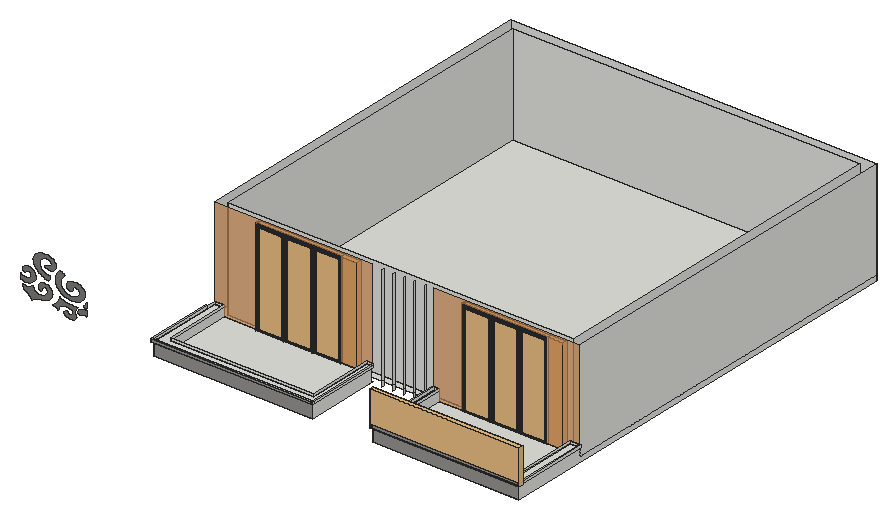
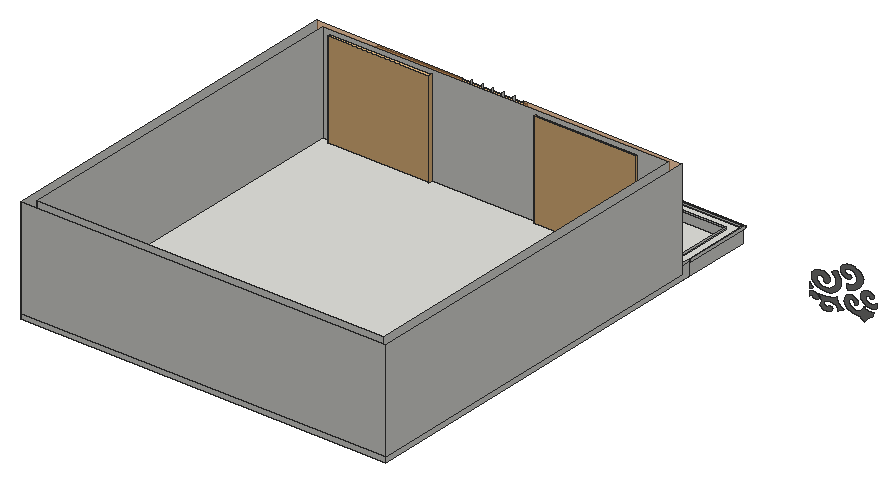
# SketchUp Ruby script. Lengths in inches.
U = 1.inch
M = Sketchup.active_model
def pt(a) = Geom::Point3d.new(a.map { |v| v * U })
def face(e, loops, mat)
  f = e.add_face(loops[0].map { |a| pt(a) })
  loops[1..].each { |l| e.add_face(l.map { |a| pt(a) }).erase! }
  f.material = f.back_material = mat if mat
  f
end
# faces: each face lists its corners as indices into pts; further lists are holes
def faces(e, pts, list, mat = nil) = list.each { |f| face(e, (f[0].is_a?(Array) ? f : [f]).map { |l| l.map { |i| pts[i] } }, mat) }
# xy, xz, yz: faces in a plane at the given z, y or x. An outline is a flat list of corners, or four numbers for a rectangle; further outlines are holes
def ring(l) = l.size == 4 ? [[l[0], l[1]], [l[2], l[1]], [l[2], l[3]], [l[0], l[3]]] : l.each_slice(2).to_a
def flat(e, list, mat, &to3) = list.each { |f| face(e, (f[0].is_a?(Array) ? f : [f]).map { |l| ring(l).map { |u, v| to3.(u, v) } }, mat) }
def xy(e, z, list, mat = nil) = flat(e, list, mat) { |x, y| [x, y, z] }
def xz(e, y, list, mat = nil) = flat(e, list, mat) { |x, z| [x, y, z] }
def yz(e, x, list, mat = nil) = flat(e, list, mat) { |y, z| [x, y, z] }
def lines(e, pts, list) = list.each { |a, b| e.add_line(pt(pts[a]), pt(pts[b])) }
# prism: a flat outline (further loops are holes) pulled along v
def prism(e, loops, v, mat = nil)
  f = face(e, loops, mat); d = Geom::Vector3d.new(v.map { |x| x * U })
  f.pushpull(f.normal.samedirection?(d) ? d.length : -d.length)
end
def box(e, o, s, mat = nil) = prism(e, [[o, [o[0] + s[0], o[1], o[2]], [o[0] + s[0], o[1] + s[1], o[2]], [o[0], o[1] + s[1], o[2]]]], [0, 0, s[2]], mat)
def at(x, y, z, deg = 0) = Geom::Transformation.translation(pt([x, y, z])) * Geom::Transformation.rotation(ORIGIN, Z_AXIS, deg.degrees)
def axes(o, x, y, z) = Geom::Transformation.new([*x, 0, *y, 0, *z, 0, *pt(o).to_a, 1])
def part(name) = M.definitions.add(name)
# library, detail: a bought-in or finely detailed component or shape, given as its bounding box
def library(name, o, s) = part(name).tap { |d| box(d.entities, o, s) }
def detail(e, o, s) = box(e.add_group.entities, o, s)
def put(e, d, t, mat = nil) = e.add_instance(d, t).tap { |i| i.material = mat if mat }
def group(e, t, mat = nil) = e.add_group.tap { |g| g.transformation = t; g.material = mat if mat }.entities
root = M.entities
M.materials.add("Wine2").color = [0, 0, 0]
M.materials["Wine2"].alpha = 0
M.materials.add("[0043_SaddleBrown]4").color = [124, 123, 122]
M.materials.add("[0130_Gainsboro]").color = [39, 45, 50]
M.materials.add("[Granite Light Gray]").color = [149, 148, 144]
M.materials.add("[Wood Floor Light]").color = [204, 176, 127]
M.materials.add("[Wood Floor]").color = [224, 152, 88]
M.materials["[Wood Floor]"].alpha = 0.68
c1 = part("Framed glazing panel")
xy(c1.entities,0,[[0,-0.98,43.07,0],[0,0,43.07,1.4]],"[0130_Gainsboro]")
xy(c1.entities,0.3,[[0.3,-1.43,42.77,-0.98]],"[0130_Gainsboro]")
xy(c1.entities,2.95,[[2.95,-1.43,40.12,-0.63],[2.95,-0.63,40.12,0],[2.95,0,40.12,0.64],[2.95,0.64,40.12,1.4]],"[0130_Gainsboro]")
xy(c1.entities,3.54,[[3.54,-0.63,39.53,0],[3.54,0,39.53,0.64]],"[0130_Gainsboro]")
xy(c1.entities,111.8125,[[3.54,-0.63,39.53,0],[3.54,0,39.53,0.64]],"[0130_Gainsboro]")
xy(c1.entities,112.4,[[2.95,-1.43,40.12,-0.63],[2.95,-0.63,40.12,0],[2.95,0,40.12,0.64],[2.95,0.64,40.12,1.4]],"[0130_Gainsboro]")
xy(c1.entities,115.05,[[0.3,-1.43,42.77,-0.98]],"[0130_Gainsboro]")
xy(c1.entities,115.35,[[0,-0.98,43.07,0],[0,0,43.07,1.4]],"[0130_Gainsboro]")
xz(c1.entities,-1.43,[[[0.3,0.3,42.77,115.05],[2.95,2.95,40.12,112.4]]],"[0130_Gainsboro]")
xz(c1.entities,-0.98,[[[0,0,43.07,115.35],[0.3,0.3,42.77,115.05]]],"[0130_Gainsboro]")
xz(c1.entities,-0.63,[[[2.95,2.95,40.12,112.4],[3.54,3.54,39.53,111.8125]]],"[0130_Gainsboro]")
xz(c1.entities,0,[[3.54,3.54,39.53,111.8125]],"Wine2")
xz(c1.entities,0,[[[0,0,43.07,115.35],[2.95,2.95,40.12,112.4]],[[2.95,2.95,40.12,112.4],[3.54,3.54,39.53,111.8125]]],"[0130_Gainsboro]")
xz(c1.entities,0.64,[[[2.95,2.95,40.12,112.4],[3.54,3.54,39.53,111.8125]]],"[0130_Gainsboro]")
xz(c1.entities,1.4,[[[0,0,43.07,115.35],[2.95,2.95,40.12,112.4]]],"[0130_Gainsboro]")
yz(c1.entities,0,[[-0.98,0,0,115.35],[0,0,1.4,115.35]],"[0130_Gainsboro]")
yz(c1.entities,0.3,[[-1.43,0.3,-0.98,115.05]],"[0130_Gainsboro]")
yz(c1.entities,2.95,[[-1.43,2.95,-0.63,112.4],[-0.63,2.95,0,112.4],[0,2.95,0.64,112.4],[0.64,2.95,1.4,112.4]],"[0130_Gainsboro]")
yz(c1.entities,3.54,[[-0.63,3.54,0,111.8125],[0,3.54,0.64,111.8125]],"[0130_Gainsboro]")
yz(c1.entities,39.53,[[-0.63,3.54,0,111.8125],[0,3.54,0.64,111.8125]],"[0130_Gainsboro]")
yz(c1.entities,40.12,[[-1.43,2.95,-0.63,112.4],[-0.63,2.95,0,112.4],[0,2.95,0.64,112.4],[0.64,2.95,1.4,112.4]],"[0130_Gainsboro]")
yz(c1.entities,42.77,[[-1.43,0.3,-0.98,115.05]],"[0130_Gainsboro]")
yz(c1.entities,43.07,[[-0.98,0,0,115.35],[0,0,1.4,115.35]],"[0130_Gainsboro]")
c2 = part("Glazing assembly")
put(c2.entities,c1,axes([90.57,1.43,0],[1.05148,0,0],[0,1,0],[0,0,1]))
put(c2.entities,c1,axes([0,1.43,0],[1.05148,0,0],[0,1,0],[0,0,1]))
put(c2.entities,c1,axes([45.29,1.43,0],[1.05148,0,0],[0,1,0],[0,0,1]))
c3 = library("Curtains",[0,0,0],[121.73,8.19,117.22])
c4 = library("Glass Railing",[0,0,0],[139.5,4.76,42])
xy(root,388.875,[[3103.26,651.03,3204.51,657.03],[3351.01,651.03,3452.26,657.03]])
xy(root,394.4375,[[3053.01,559.875,3243.69,570.83],[3316.14,559.875,3491.44,570.83],[3064.33,657.03,3480.11,1085.17]])
xy(root,394.4375,[[3053.01,570.83,3064.33,651.03],[3064.33,570.83,3243.69,651.03],[3316.14,570.83,3480.11,651.03],[3480.11,570.83,3491.44,651.03]],"[Wood Floor Light]")
xy(root,400.4375,[[3064.33,570.83,3235.84,570.83,3235.84,651.03,3204.51,651.03,3204.51,657.03,3103.26,657.03,3103.26,651.03,3064.33,651.03],[3322.22,570.83,3480.11,570.83,3480.11,651.03,3452.26,651.03,3452.26,657.03,3351.01,657.03,3351.01,651.03,3322.22,651.03],[3053.01,651.03,3053.01,1096.5,3491.44,1096.5,3491.44,651.03,3452.26,651.03,3452.26,657.03,3480.11,657.03,3480.11,1085.17,3064.33,1085.17,3064.33,657.03,3103.26,657.03,3103.26,651.03],[3064.33,657.03,3480.11,1085.17]])
xy(root,410.625,[[3051.26,557.9375,3243.69,559.875],[3243.69,557.9375,3245.63,559.875],[3314.21,557.9375,3316.14,559.875],[3316.14,557.9375,3491.44,559.875],[3491.44,557.9375,3493.37,559.875],
  [3051.07,559.875,3053.01,640.11],[3053.01,559.875,3053.01,651.03,3064.33,651.03,3064.33,570.83,3235.84,570.83,3235.84,651.03,3243.69,651.03,3243.69,559.875],[3243.69,559.875,3245.63,647.91],[3314.21,559.875,3316.14,651.03],[3316.14,559.875,3316.14,651.03,3322.22,651.03,3322.22,570.83,3480.11,570.83,3480.11,651.03,3491.44,651.03,3491.44,559.875],
  [3491.44,559.875,3493.37,651.03]])
xz(root,557.9375,[[3491.44,410.625,3493.37,413.5]])
xz(root,557.9375,[[3051.26,410.625,3243.69,413.5],[3243.69,410.625,3245.63,413.5],[3314.21,410.625,3316.14,413.5],[3316.14,410.625,3491.44,413.5]],"[Granite Light Gray]")
xz(root,559.875,[[3051.07,410.625,3051.26,413.5],[3051.26,410.625,3053.01,413.5],[3053.01,410.625,3243.69,413.5],[3243.69,410.625,3245.63,413.5],[3314.21,410.625,3316.14,413.5],
  [3316.14,410.625,3491.44,413.5],[3491.44,410.625,3493.37,413.5]])
xz(root,559.875,[[3053.01,394.4375,3243.69,410.625],[3316.14,394.4375,3491.44,410.625]],"[Granite Light Gray]")
xz(root,570.83,[[3064.33,400.4375,3235.84,410.625],[3322.22,400.4375,3480.11,410.625],[3064.33,410.625,3235.84,413.5],[3322.22,410.625,3480.11,413.5]])
xz(root,589.17,[[2928.78,378.34,2930.4375,378.37,2932.06,378.64,2933.5625,379.15,2934.89,379.86,2935.99,380.76,2936.81,381.8,2936.25,382.74,2935.8,383.71,2935.48,384.71,2935.28,385.72,2935.2,386.75,2935.25,387.77,2935.43,388.79,2935.73,389.79,2936.15,390.76,2936.69,391.71,2937.35,392.62,2938.11,393.48,2936.23,393.37,2934.35,393.33,2932.46,393.38,2930.59,393.5,2928.72,393.71,2926.88,393.99,2925.06,394.35,2923.27,394.79,2921.53,395.3,2919.82,395.88,2918.17,396.54,2916.57,397.26,2916.46,396.19,2916.23,395.13,2915.89,394.09,2915.44,393.07,2914.89,392.07,2914.24,391.11,2913.49,390.1875,2912.64,389.31,2911.71,388.47,2910.6875,387.69,2909.59,386.97,2908.42,386.31,2909.04,386.1,2909.65,385.89,2910.26,385.67,2910.86,385.44,2911.45,385.2,2912.04,384.95,2912.62,384.7,2913.19,384.44,2913.75,384.16,2914.3125,383.88,2914.86,383.59,2915.4,383.3,2915.51,384.7,2916.03,386.05,2916.95,387.29,2918.23,388.35,2919.79,389.19,2921.57,389.77,2923.47,390.05,2925.42,390.03,2927.32,389.7,2929.07,389.08,2930.59,388.2,2931.81,387.11,2931.85,386.77,2931.87,386.43,2931.87,385.75,2931.81,385.07,2931.76,384.73,2931.69,384.39,2931.61,384.06,2931.52,383.72,2931.42,383.39,2931.29,383.06,2930.7,382.875,2930.07,382.76,2929.43,382.72,2928.78,382.75,2928.15,382.85,2927.55,383.03,2927,383.27,2926.5,383.58,2926.08,383.93,2925.75,384.33,2925.5,384.76,2925.36,385.22,2924.95,385.09,2924.5625,384.95,2924.18,384.79,2923.82,384.61,2923.47,384.41,2923.14,384.2,2922.83,383.98,2922.53,383.74,2922.26,383.48,2922.02,383.22,2921.79,382.95,2921.59,382.66,2922.18,381.54,2923.07,380.53,2924.23,379.68,2925.61,379.01,2927.14,378.55],[2883.21,382.25,2883.82,383.03,2884.54,383.77,2885.35,384.44,2886.26,385.06,2887.25,385.6,2888.3125,386.07,2889.44,386.46,2890.61,386.77,2891.82,386.98,2893.05,387.11,2894.29,387.15,2895.54,387.09,2897.95,387.5,2900.24,388.2,2902.32,389.18,2904.125,390.4,2905.61,391.84,2906.73,393.4375,2907.44,395.15,2907.73,396.93,2907.58,398.71,2907.01,400.46,2906.02,402.1,2904.65,403.59,2903.52,404.41,2902.18,405.05,2900.68,405.47,2899.09,405.65,2897.49,405.59,2895.9375,405.29,2894.51,404.75,2893.27,404.02,2892.27,403.11,2891.56,402.07,2891.16,400.95,2891.11,399.79,2891.17,399.43,2891.28,399.08,2891.44,398.73,2891.65,398.4,2891.91,398.09,2892.21,397.8,2892.55,397.53,2892.92,397.29,2893.33,397.08,2893.77,396.9,2894.23,396.75,2894.71,396.64,2894.79,397.15,2894.91,397.65,2895.07,398.15,2895.28,398.64,2895.52,399.13,2895.8,399.6,2896.12,400.06,2896.48,400.5,2896.87,400.93,2897.29,401.34,2897.75,401.74,2898.24,402.11,2899.17,401.77,2900.02,401.34,2900.77,400.81,2901.4,400.2,2901.89,399.54,2902.23,398.83,2902.42,398.08,2902.44,397.33,2902.3,396.58,2902.01,395.86,2901.57,395.18,2900.98,394.55,2900.14,393.61,2899.07,392.8,2897.82,392.14,2896.42,391.66,2894.92,391.38,2893.37,391.3,2891.83,391.43,2890.34,391.76,2888.97,392.28,2887.76,392.98,2886.74,393.82,2885.96,394.79,2885.74,395.05,2885.54,395.3125,2885.35,395.58,2885.17,395.85,2885,396.13,2884.85,396.41,2884.71,396.69,2884.58,396.98,2884.47,397.27,2884.36,397.5625,2884.27,397.86,2884.2,398.15,2883.51,397.49,2882.71,396.89,2881.81,396.375,2880.83,395.94,2879.78,395.6,2878.6875,395.35,2877.55,395.2,2876.41,395.16,2875.26,395.22,2874.13,395.38,2873.04,395.64,2872,396,2872.22,395.6875,2872.41,395.37,2872.57,395.04,2872.71,394.71,2872.83,394.375,2872.91,394.03,2872.97,393.6875,2873,393.34,2873.01,392.99,2872.98,392.65,2872.93,392.3,2872.85,391.96,2874,391.33,2875.09,390.67,2876.15,389.96,2877.15,389.22,2878.11,388.45,2879.01,387.64,2879.86,386.81,2880.65,385.95,2881.38,385.06,2882.05,384.14,2882.66,383.2],[2941.32,386.82,2941.86,386.85,2942.32,386.92,2942.78,387.02,2943.21,387.15,2943.63,387.31,2944.03,387.49,2944.41,387.7,2944.76,387.93,2945.08,388.18,2945.36,388.45,2945.61,388.74,2945.83,389.05,2946.01,389.36,2946.35,389.23,2946.6875,389.09,2947.02,388.93,2947.34,388.77,2947.66,388.6,2947.97,388.43,2948.27,388.24,2948.56,388.05,2948.84,387.85,2949.11,387.65,2949.37,387.4375,2949.62,387.22,2949.62,393,2948.64,393.38,2947.6,393.65,2946.51,393.8,2945.4,393.8125,2944.3,393.7,2943.24,393.47,2942.24,393.11,2941.34,392.65,2940.55,392.09,2939.89,391.45,2939.38,390.73,2939.04,389.97,2938.78,389.63,2938.625,389.25,2938.57,388.86,2938.62,388.47,2938.78,388.09,2939.03,387.74,2939.37,387.4375,2939.78,387.18,2940.26,386.99,2940.78,386.87],[2949.23,396.46,2949.62,396.47,2949.62,402.56,2949.34,402.125,2949.04,401.6875,2948.74,401.26,2948.42,400.83,2948.09,400.41,2947.75,399.99,2947.4,399.58,2947.04,399.18,2946.66,398.77,2946.28,398.38,2945.88,397.99,2945.47,397.61,2945.75,397.42,2946.04,397.24,2946.35,397.08,2946.68,396.9375,2947.02,396.8125,2947.37,396.71,2947.73,396.62,2948.1,396.55,2948.47,396.5,2948.85,396.47],[2931.11,398.78,2933.31,398.88,2935.48,399.21,2937.56,399.74,2939.52,400.47,2941.32,401.39,2942.94,402.47,2944.33,403.7,2945.48,405.0625,2946.36,406.52,2946.96,408.05,2947.27,409.625,2947.26,410.99,2946.98,412.35,2946.43,413.65,2945.61,414.89,2944.56,416.03,2943.29,417.04,2941.82,417.91,2940.19,418.61,2938.44,419.14,2936.6,419.47,2934.72,419.61,2932.82,419.54,2931.35,419.33,2929.94,418.9375,2928.65,418.39,2927.49,417.7,2926.51,416.875,2925.73,415.95,2925.17,414.95,2924.84,413.89,2924.76,412.81,2924.93,411.73,2925.34,410.68,2925.98,409.7,2926.49,409.31,2927.11,409,2927.8,408.79,2928.54,408.68,2929.29,408.6875,2930.02,408.8,2930.71,409.03,2931.32,409.35,2931.82,409.75,2932.2,410.22,2932.43,410.73,2932.32,411.09,2932.26,411.45,2932.26,411.81,2932.3125,412.17,2932.42,412.52,2932.59,412.87,2932.8,413.19,2933.07,413.5,2933.38,413.79,2933.73,414.04,2934.125,414.27,2934.55,414.46,2935.56,414.36,2936.54,414.15,2937.46,413.83,2938.3,413.41,2939.04,412.9,2939.66,412.32,2940.16,411.68,2940.51,410.98,2940.71,410.26,2940.75,409.53,2940.64,408.8,2940.37,408.08,2939.62,406.9,2938.61,405.82,2937.36,404.88,2935.92,404.1,2934.3125,403.5,2932.59,403.11,2930.8,402.93,2929,402.96,2927.23,403.22,2925.54,403.68,2923.98,404.34,2922.6,405.17,2921.15,406.36,2919.92,407.66,2918.95,409.08,2918.24,410.57,2917.8125,412.12,2917.67,413.7,2917.8125,415.27,2918.24,416.82,2918.95,418.3125,2919.92,419.73,2921.15,421.04,2922.6,422.22,2922.23,422.57,2921.85,422.9,2921.44,423.22,2921.02,423.53,2920.58,423.82,2920.11,424.1,2919.63,424.37,2919.14,424.61,2918.63,424.84,2918.1,425.06,2917.57,425.25,2917.02,425.43,2915.89,424.36,2914.88,423.23,2913.99,422.04,2913.23,420.8125,2912.59,419.55,2912.09,418.25,2911.72,416.93,2911.49,415.6,2911.4,414.25,2911.44,412.91,2911.625,411.57,2911.95,410.24,2912.48,408.8125,2913.21,407.43,2914.13,406.1,2915.23,404.85,2916.51,403.69,2917.94,402.63,2919.51,401.68,2921.22,400.85,2923.02,400.15,2924.92,399.58,2926.89,399.16,2928.91,398.88],
  [2876.22,399.74,2877.3,399.78,2878.36,399.9,2879.4,400.1,2880.42,400.36,2881.39,400.7,2883.08,401.49,2884.58,402.47,2885.84,403.61,2886.83,404.88,2887.53,406.25,2887.91,407.68,2887.97,409.14,2887.71,410.58,2887.13,411.98,2886.24,413.29,2885.08,414.48,2883.67,415.52,2882.6875,416.12,2881.57,416.58,2880.35,416.875,2879.08,417,2877.8,416.95,2876.55,416.72,2875.38,416.33,2874.34,415.79,2873.46,415.12,2872.77,414.34,2872.29,413.48,2872.05,412.57,2871.96,412.22,2871.97,411.86,2872.07,411.51,2872.26,411.18,2872.54,410.89,2872.9,410.63,2873.31,410.4375,2873.77,410.3,2874.25,410.24,2874.75,410.24,2875.24,410.31,2875.69,410.45,2875.96,410.7,2876.25,410.9375,2876.56,411.17,2876.89,411.38,2877.23,411.58,2877.6,411.76,2877.97,411.92,2878.37,412.07,2878.77,412.2,2879.18,412.31,2879.61,412.4,2880.03,412.47,2880.6,412.12,2881.1,411.73,2881.53,411.29,2881.875,410.82,2882.15,410.32,2882.33,409.8,2882.42,409.27,2882.42,408.74,2882.33,408.2,2882.15,407.69,2881.89,407.1875,2881.54,406.71,2880.8125,406,2879.93,405.39,2878.91,404.89,2877.79,404.53,2876.61,404.3,2875.38,404.23,2874.16,404.3,2872.97,404.53,2871.85,404.89,2870.84,405.39,2869.95,406,2869.23,406.71,2869.23,401.47,2870.1,401.01,2871.03,400.625,2872.01,400.3,2873.03,400.05,2874.08,399.875,2875.15,399.77],[2903.25,409.96,2903.66,410.4,2904.03,410.87,2904.34,411.35,2904.6,411.86,2904.8125,412.37,2904.97,412.89,2905.07,413.42,2905.11,413.96,2905.1,414.49,2905.04,415.03,2904.92,415.56,2904.74,416.08,2903.39,415.96,2902.03,415.98,2900.69,416.14,2899.38,416.43,2898.15,416.85,2897.01,417.38,2895.98,418.02,2895.08,418.76,2894.34,419.58,2893.76,420.47,2893.35,421.4,2893.125,422.37,2892.76,423.29,2892.53,424.22,2892.4375,425.17,2892.49,426.125,2892.68,427.06,2893.02,427.99,2893.48,428.875,2894.08,429.73,2894.8,430.52,2895.63,431.26,2896.57,431.93,2897.6,432.53,2898.56,432.92,2899.6,433.1875,2900.7,433.3,2901.8,433.26,2902.875,433.08,2903.88,432.75,2904.79,432.29,2905.55,431.71,2906.15,431.04,2906.57,430.3,2906.78,429.52,2906.78,428.72,2906.7,428.33,2906.54,427.95,2906.31,427.59,2906.01,427.25,2905.65,426.95,2905.24,426.6875,2904.78,426.46,2904.29,426.29,2903.76,426.16,2903.22,426.09,2902.67,426.07,2902.12,426.11,2901.55,426.125,2900.98,426.05,2900.46,425.88,2900,425.63,2899.63,425.3125,2899.37,424.94,2899.24,424.54,2899.23,424.13,2899.36,423.72,2899.61,423.35,2899.97,423.03,2900.42,422.77,2901.66,422.33,2903,422.0625,2904.39,421.97,2905.77,422.0625,2907.11,422.33,2908.35,422.77,2909.47,423.37,2910.41,424.1,2911.16,424.95,2911.68,425.875,2911.96,426.86,2911.98,427.86,2912.04,429.07,2911.86,430.28,2911.46,431.45,2910.83,432.58,2910,433.63,2908.98,434.59,2907.78,435.44,2906.43,436.17,2904.95,436.75,2903.38,437.18,2901.74,437.46,2900.07,437.5625,2897.73,437.47,2895.45,437.11,2893.27,436.49,2891.25,435.64,2889.4375,434.58,2887.88,433.32,2886.61,431.9,2885.67,430.36,2885.07,428.73,2884.83,427.05,2884.96,425.37,2885.45,423.72,2886,422.12,2886.76,420.56,2887.71,419.06,2888.85,417.63,2890.16,416.28,2891.65,415.02,2893.28,413.87,2895.06,412.83,2896.96,411.91,2898.97,411.12,2901.07,410.47]],"[0043_SaddleBrown]4")
xz(root,640.11,[[3051.07,410.625,3053.01,413.5]])
xz(root,647.91,[[3243.69,410.625,3245.63,413.5]])
xz(root,651.03,[[3053.01,400.4375,3064.33,410.625],[3480.11,400.4375,3491.44,410.625],[3053.01,410.625,3064.33,413.5],[3235.84,410.625,3243.69,413.5],[3314.21,410.625,3315.93,413.5],
  [3315.93,410.625,3316.14,413.5],[3316.14,410.625,3322.22,413.5],[3480.11,410.625,3491.44,413.5],[3491.44,410.625,3493.37,413.5]])
xz(root,651.03,[[3064.33,400.4375,3103.26,400.4375,3103.26,514.875,3204.51,514.875,3204.51,400.4375,3235.84,400.4375,3235.84,413.5,3243.69,413.5,3243.69,520.4375,3053.01,520.4375,3053.01,413.5,3064.33,413.5],[3322.22,400.4375,3351.01,400.4375,3351.01,514.875,3452.26,514.875,3452.26,400.4375,3480.11,400.4375,3480.11,413.5,3491.44,413.5,3491.44,520.4375,3316.14,520.4375,3316.14,413.5,3322.22,413.5]],"[Wood Floor]")
xz(root,657.03,[[3064.33,400.4375,3064.33,520.4375,3480.11,520.4375,3480.11,400.4375,3452.26,400.4375,3452.26,514.875,3351.01,514.875,3351.01,400.4375,3204.51,400.4375,3204.51,514.875,3103.26,514.875,3103.26,400.4375]])
xz(root,1085.17,[[3064.33,400.4375,3480.11,520.4375]])
xz(root,1096.5,[[3053.01,394.4375,3491.44,400.4375],[3053.01,400.4375,3491.44,520.4375]])
yz(root,3051.07,[[559.875,410.625,640.11,413.5]])
yz(root,3051.26,[[557.9375,410.625,559.875,413.5]])
yz(root,3053.01,[[559.875,394.4375,640.11,410.625],[640.11,394.4375,640.11,410.625,651.03,410.625,651.03,400.4375,1096.5,400.4375,1096.5,394.4375],[651.03,400.4375,1096.5,520.4375],[559.875,410.625,640.11,413.5],[640.11,410.625,651.03,413.5]])
yz(root,3064.33,[[570.83,400.4375,651.03,410.625],[657.03,400.4375,1085.17,520.4375],[570.83,410.625,651.03,413.5]])
yz(root,3103.26,[[651.03,400.4375,657.03,514.875]])
yz(root,3204.51,[[651.03,400.4375,657.03,514.875]])
yz(root,3235.84,[[570.83,400.4375,651.03,410.625],[570.83,410.625,651.03,413.5]])
yz(root,3243.69,[[559.875,394.4375,647.91,410.625],[557.9375,410.625,559.875,413.5],[559.875,410.625,647.91,413.5],[647.91,410.625,651.03,413.5]])
yz(root,3245.63,[[557.9375,410.625,559.875,413.5],[559.875,410.625,647.91,413.5]])
yz(root,3256.69,[[647.91,394.4375,651.03,400.4375],[647.91,400.4375,651.03,520.4375]])
yz(root,3269.44,[[648.85,394.4375,651.03,400.4375],[648.85,400.4375,651.03,520.4375]])
yz(root,3281.57,[[648.85,394.4375,651.03,400.4375],[648.85,400.4375,651.03,520.4375]])
yz(root,3293.94,[[648.85,394.4375,651.03,400.4375],[648.85,400.4375,651.03,520.4375]])
yz(root,3306.82,[[648.85,394.4375,651.03,400.4375],[648.85,400.4375,651.03,520.4375]])
yz(root,3314.21,[[557.9375,410.625,559.875,413.5],[559.875,410.625,651.03,413.5]])
yz(root,3316.14,[[559.875,394.4375,651.03,410.625],[557.9375,410.625,559.875,413.5],[559.875,410.625,651.03,413.5]])
yz(root,3322.22,[[570.83,400.4375,651.03,410.625],[570.83,410.625,651.03,413.5]])
yz(root,3351.01,[[651.03,400.4375,657.03,514.875]])
yz(root,3452.26,[[651.03,400.4375,657.03,514.875]])
yz(root,3480.11,[[570.83,400.4375,651.03,410.625],[657.03,400.4375,1085.17,520.4375],[570.83,410.625,651.03,413.5]])
yz(root,3491.44,[[559.875,394.4375,1096.5,394.4375,1096.5,400.4375,651.03,400.4375,651.03,410.625,559.875,410.625],[651.03,400.4375,1096.5,520.4375],[557.9375,410.625,559.875,413.5],[559.875,410.625,651.03,413.5]])
yz(root,3493.37,[[557.9375,410.625,559.875,413.5],[559.875,410.625,651.03,413.5]])
p = [[2932.52,589.17,411.27],[2932.43,589.17,410.73]]
lines(root,p,[[0,1]])
put(root,c2,axes([3102.86,650.7,397.79],[0.75,0,0],[0,0.75,0],[0,0,1.01765]))
put(root,c3,at(3102.07,651.68,397.95))
put(root,c2,axes([3350.36,651.03,397.48],[0.75,0,0],[0,0.75,0],[0,0,1.01765]))
put(root,c4,axes([3314.21,558.12,409.93],[1.28434,0,0],[0,1,0],[0,0,1]),"[Granite Light Gray]")
put(root,c3,at(3349.11,652.22,397.95))
